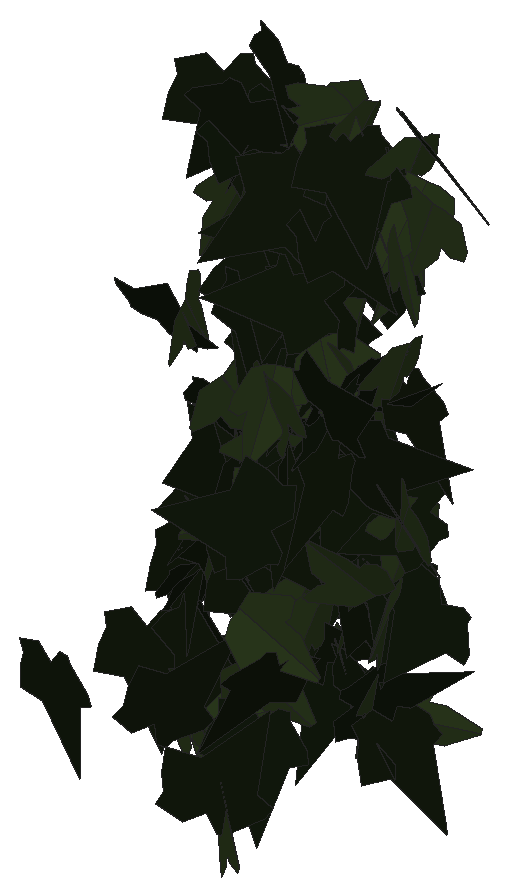
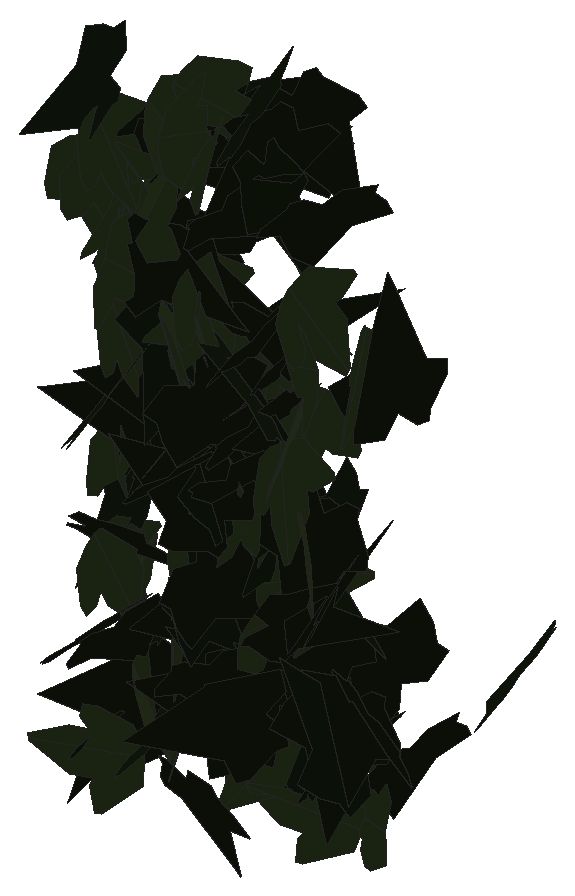
# SketchUp Ruby script. Lengths in inches.
U = 1.inch
M = Sketchup.active_model
def pt(a) = Geom::Point3d.new(a.map { |v| v * U })
def face(e, loops, mat)
  f = e.add_face(loops[0].map { |a| pt(a) })
  loops[1..].each { |l| e.add_face(l.map { |a| pt(a) }).erase! }
  f.material = f.back_material = mat if mat
  f
end
# faces: each face lists its corners as indices into pts; further lists are holes
def faces(e, pts, list, mat = nil) = list.each { |f| face(e, (f[0].is_a?(Array) ? f : [f]).map { |l| l.map { |i| pts[i] } }, mat) }
# xy, xz, yz: faces in a plane at the given z, y or x. An outline is a flat list of corners, or four numbers for a rectangle; further outlines are holes
def ring(l) = l.size == 4 ? [[l[0], l[1]], [l[2], l[1]], [l[2], l[3]], [l[0], l[3]]] : l.each_slice(2).to_a
def flat(e, list, mat, &to3) = list.each { |f| face(e, (f[0].is_a?(Array) ? f : [f]).map { |l| ring(l).map { |u, v| to3.(u, v) } }, mat) }
def xy(e, z, list, mat = nil) = flat(e, list, mat) { |x, y| [x, y, z] }
def xz(e, y, list, mat = nil) = flat(e, list, mat) { |x, z| [x, y, z] }
def yz(e, x, list, mat = nil) = flat(e, list, mat) { |y, z| [x, y, z] }
def lines(e, pts, list) = list.each { |a, b| e.add_line(pt(pts[a]), pt(pts[b])) }
# prism: a flat outline (further loops are holes) pulled along v
def prism(e, loops, v, mat = nil)
  f = face(e, loops, mat); d = Geom::Vector3d.new(v.map { |x| x * U })
  f.pushpull(f.normal.samedirection?(d) ? d.length : -d.length)
end
def box(e, o, s, mat = nil) = prism(e, [[o, [o[0] + s[0], o[1], o[2]], [o[0] + s[0], o[1] + s[1], o[2]], [o[0], o[1] + s[1], o[2]]]], [0, 0, s[2]], mat)
def at(x, y, z, deg = 0) = Geom::Transformation.translation(pt([x, y, z])) * Geom::Transformation.rotation(ORIGIN, Z_AXIS, deg.degrees)
def axes(o, x, y, z) = Geom::Transformation.new([*x, 0, *y, 0, *z, 0, *pt(o).to_a, 1])
def part(name) = M.definitions.add(name)
# library, detail: a bought-in or finely detailed component or shape, given as its bounding box
def library(name, o, s) = part(name).tap { |d| box(d.entities, o, s) }
def detail(e, o, s) = box(e.add_group.entities, o, s)
def put(e, d, t, mat = nil) = e.add_instance(d, t).tap { |i| i.material = mat if mat }
def group(e, t, mat = nil) = e.add_group.tap { |g| g.transformation = t; g.material = mat if mat }.entities
root = M.entities
M.materials.add("efeu1").color = [18, 25, 13]
M.materials.add("efeu2").color = [43, 57, 29]
c1 = part("ivyleaf_9")
p = [[1.54,2.16,1.25],[1.36,2.04,1.19],[-0.21,0.99,0.68],[-0.71,1.11,0.82],[-0.85,0.86,0.67],[-0.8,0.17,0.21],
  [-0.9,-0.01,0.1],[-0.67,-0.16,-0.02],[-0.08,-0.08,-0.05],[-0.03,-0.6,-0.4],[0.65,-0.88,-0.66],[0.83,-0.6,-0.49],
  [1.29,-0.42,-0.43],[1.8125,-0.07,-0.26],[1.21,0.44,0.15]]
faces(c1.entities,p,[[0,1,2,3,4,5,6,7,8,9,10,11,12,13,14]],"efeu1")
c2 = part("ivyleaf_10")
p = [[0,0.5,-0.03],[-0.0625,2.02,-0.43],[-0.19,2.01,-0.46],[-0.54,1.05,-0.29],[-0.52,0.625,-0.18],[-0.83,0.76,-0.28],
  [-1.16,0.64,-0.33],[-1.15,0.33,-0.24],[-0.77,-0.39,0.02],[-0.3,-0.51,0.16],[0.04,-0.48,0.23],[-0.02,2.01,-0.4375],
  [-0.06,2.01,-0.43],[0.04,-0.49,0.23],[0.67,-0.49,0.14],[1.38,0.36,-0.2],[1.375,0.51,-0.24],[0.81,0.65,-0.19],
  [0.62,0.59,-0.15],[0.6,1.09,-0.28],[0.5,1.23,-0.31]]
faces(c2.entities,p,[[0,1,2,3,4,5,6,7,8,9,10],[11,12,0,13,14,15,16,17,18,19,20]],"efeu2")
put(root,c1,axes([39.76,218.64,235.83],[-0.13606,0.27055,-0.39786],[0.04668,-0.40409,-0.29075],[-0.47886,-0.11626,0.0847]))
put(root,c1,axes([36.25,218.75,234.58],[0.18702,-0.45521,0.08836],[0.03479,-0.08123,-0.49213],[0.4624,0.19023,0.00129]))
put(root,c1,axes([39.43,218.87,237.54],[-0.20466,-0.00713,0.45614],[-0.39206,-0.25286,-0.17986],[0.23324,-0.43129,0.09792]))
put(root,c2,axes([38.78,218.87,233.33],[0.01309,-0.03717,0.49844],[0.43605,-0.24288,-0.02956],[0.24432,0.43546,0.02605]))
put(root,c2,axes([39.38,218.69,236.29],[0.21409,0.09828,0.44103],[0.40366,0.1777,-0.23555],[-0.20304,0.45691,-0.00325]))
put(root,c1,axes([38.51,218.92,233.37],[-0.26224,-0.03724,0.42408],[0.42523,0.00076,0.26302],[-0.02024,0.49861,0.03127]))
put(root,c1,axes([37.61,219.08,234.19],[-0.04947,-0.09741,0.48792],[0.43073,0.23704,0.091],[-0.24904,0.42933,0.06046]))
put(root,c1,axes([39.52,219.89,238.75],[0.00714,-0.088,0.49214],[0.33503,-0.36449,-0.07004],[0.37109,0.33076,0.05376]))
put(root,c1,axes([39.68,219.88,238.1],[-0.44399,0.06238,-0.22132],[0.21925,-0.0302,-0.44835],[-0.06931,-0.49517,-0.00053]))
put(root,c2,axes([39.91,220.1,236.36],[-0.40421,-0.08589,-0.28149],[-0.23076,-0.20433,0.3937],[-0.18266,0.44819,0.12554]))
put(root,c1,axes([37.66,220.07,236.33],[0.2605,-0.32329,0.27862],[0.18678,-0.20714,-0.41498],[0.38374,0.32028,0.01285]))
put(root,c1,axes([38.71,220.39,241.16],[-0.31078,-0.28387,0.26988],[-0.20949,-0.17063,-0.42071],[0.33095,-0.37457,-0.01288]))
put(root,c1,axes([38.23,220.25,233.8],[-0.06334,-0.49315,-0.05281],[0.00648,0.05242,-0.4972],[0.49593,-0.06367,-0.00025]))
put(root,c2,axes([38.35,220.33,238.47],[0.17904,0.42174,-0.20019],[-0.09684,-0.17619,-0.4578],[-0.45669,0.2027,0.01859]))
put(root,c1,axes([38.63,220.4375,237.36],[-0.349,-0.18893,-0.30415],[0.32579,0.00863,-0.37919],[0.14853,-0.46285,0.11707]))
put(root,c1,axes([36.36,220.42,234.37],[0.01984,-0.48648,-0.11377],[-0.01924,0.11303,-0.48668],[0.49924,0.02369,-0.01423]))
put(root,c1,axes([38.87,220.58,239.74],[-0.29959,-0.02659,0.39942],[-0.33646,-0.25359,-0.26924],[0.2169,-0.4301,0.13405]))
put(root,c1,axes([39.4,220.11,238.43],[-0.17276,0.42988,0.18803],[-0.08534,0.16824,-0.46305],[-0.46138,-0.19209,0.01525]))
put(root,c2,axes([38.4,220.3,238.44],[-0.45879,0.17255,0.09869],[-0.09876,0.01757,-0.48983],[-0.17251,-0.46895,0.01796]))
put(root,c1,axes([37.99,220.3,236.6875],[-0.05967,-0.17832,-0.46329],[0.17798,0.42792,-0.18763],[0.46343,-0.1873,0.0124]))
put(root,c2,axes([36.67,220.59,233.44],[0.02179,-0.1026,0.48887],[0.48921,-0.09452,-0.04165],[0.10097,0.48014,0.09627]))
put(root,c1,axes([38.72,220.76,240.77],[-0.31497,-0.10729,0.37321],[-0.32879,-0.182,-0.32981],[0.20662,-0.45317,0.0441]))
put(root,c1,axes([36.375,220.64,238.58],[0.49365,-0.07686,-0.02004],[0.02026,-0.00015,0.49959],[-0.0768,-0.49406,0.00297]))
put(root,c2,axes([39.67,220.93,235.59],[-0.13396,0.02209,-0.48121],[0.10821,-0.48533,-0.0524],[-0.46941,-0.11818,0.12525]))
put(root,c1,axes([36.93,220.95,234.24],[-0.09406,-0.44669,0.204],[-0.002,-0.20736,-0.45497],[0.49107,-0.0864,0.03722]))
put(root,c1,axes([37.76,220.71,235.64],[0.04044,-0.47239,-0.15879],[-0.01342,0.15822,-0.47412],[0.49818,0.04261,0.00012]))
put(root,c2,axes([38.54,220.85,235.16],[0.0001,-0.4324,0.25106],[0.07571,-0.24815,-0.42742],[0.49423,0.0381,0.06543]))
put(root,c1,axes([37.13,220.92,234.2],[0.05501,-0.20512,0.45266],[0.24457,-0.38528,-0.20431],[0.43262,0.24389,0.05794]))
put(root,c2,axes([38.18,220.67,237.43],[-0.41792,-0.26691,0.06405],[-0.04939,-0.04166,-0.49581],[0.27001,-0.42074,0.00846]))
put(root,c2,axes([37.63,221,236.17],[0.00677,-0.02501,0.49933],[-0.15615,-0.4745,-0.02164],[0.47494,-0.15565,-0.01423]))
put(root,c2,axes([36.9,220.51,238.99],[0.12288,-0.38521,-0.29414],[0.02475,0.30804,-0.39307],[0.48403,0.08204,0.09477]))
put(root,c1,axes([37.63,220.77,241.88],[0.14433,0.19089,-0.43901],[-0.24233,-0.36631,-0.23894],[-0.41285,0.28174,-0.01322]))
put(root,c2,axes([37.52,220.58,238.09],[-0.20547,-0.37433,-0.26011],[0.16813,0.20296,-0.4249],[0.42369,-0.26207,0.04247]))
put(root,c2,axes([37.41,220.41,235.96],[0.07698,-0.16348,-0.4662],[-0.00652,0.47145,-0.1664],[0.494,0.0317,0.07046]))
put(root,c1,axes([38.92,220.68,240.84],[0.21776,-0.3615,-0.26813],[-0.03657,0.28267,-0.4108],[0.4486,0.19853,0.09667]))
put(root,c1,axes([38.96,221.11,235.5],[0.04763,-0.30648,0.39217],[0.08264,-0.38362,-0.30984],[0.49082,0.09434,0.01411]))
put(root,c2,axes([37.17,220.625,233.3],[0.18953,-0.03808,-0.46111],[0.45175,0.12291,0.17554],[0.09998,-0.48316,0.081]))
put(root,c1,axes([37.37,220.88,236.59],[-0.40634,0.24107,-0.16361],[0.11579,-0.12404,-0.47033],[-0.26735,-0.42012,0.04498]))
put(root,c2,axes([38.86,220.72,238.85],[0.16076,0.46841,0.0689],[0.01678,0.06708,-0.4952],[-0.47315,0.16153,0.00585]))
put(root,c1,axes([39.03,221.15,237.29],[-0.11335,-0.46483,0.1452],[-0.03646,-0.14056,-0.47845],[0.48562,-0.11905,-0.00203]))
put(root,c1,axes([38.5,221,238.58],[-0.4439,0.06429,-0.22096],[0.20999,-0.08323,-0.44607],[-0.09414,-0.48881,0.04689]))
put(root,c1,axes([38.42,220.54,237.43],[0.16874,-0.01161,-0.47052],[-0.39558,0.26734,-0.14846],[0.25503,0.42236,0.08104]))
put(root,c1,axes([37.51,221.12,238.98],[0.06689,-0.48049,0.12108],[0.0066,-0.1213,-0.48502],[0.49546,0.06649,-0.00989]))
put(root,c2,axes([38.14,221.11,235.16],[-0.05033,-0.42618,0.25659],[0.04615,-0.26079,-0.4241],[0.49531,-0.01901,0.06559]))
put(root,c1,axes([37.65,221.1,236.71],[0.24905,-0.30701,0.30614],[0.17873,-0.24896,-0.39506],[0.395,0.30622,-0.01426]))
put(root,c2,axes([37.75,220.78,234.16],[-0.35852,-0.17582,-0.30092],[0.27155,0.12969,-0.3993],[0.21846,-0.44974,0.0025]))
put(root,c1,axes([38.41,220.9,237.67],[-0.39828,0.30186,-0.01598],[0.01187,-0.01079,-0.49974],[-0.30205,-0.39845,0.00143]))
put(root,c1,axes([37.375,220.79,235.7],[0.27858,0.3249,-0.25852],[-0.17991,-0.18612,-0.42778],[-0.3742,0.33136,0.01321]))
put(root,c1,axes([37.66,221.14,239.4],[-0.37858,-0.26699,-0.18813],[0.15865,0.10142,-0.46319],[0.28549,-0.4104,0.00792]))
put(root,c1,axes([39.18,220.64,238.6],[0.11541,0.46581,0.14036],[0.03415,0.13614,-0.47989],[-0.4853,0.12035,-0.00039]))
put(root,c2,axes([39.35,221.14,234.4375],[0.22315,-0.43437,0.10734],[0.03799,-0.10112,-0.48819],[0.44582,0.22604,-0.01212]))
put(root,c2,axes([38.68,220.93,238.83],[-0.45257,0.03297,0.20999],[-0.2084,0.02845,-0.45361],[-0.04186,-0.4981,-0.01201]))
put(root,c1,axes([38.84,221.02,239.51],[-0.22718,-0.00558,-0.44537],[-0.40969,-0.19354,0.21141],[-0.17476,0.46099,0.08337]))
put(root,c2,axes([38.93,220.83,237.95],[0.20368,-0.3132,-0.33229],[-0.05946,0.34256,-0.35933],[0.45274,0.1859,0.1023]))
put(root,c1,axes([38.89,221.17,241.58],[-0.0484,-0.47345,-0.1533],[0.03336,0.15059,-0.47561],[0.49653,-0.05627,0.01701]))
put(root,c1,axes([36.71,221.4375,236.34],[-0.13244,-0.15306,0.4572],[-0.09101,-0.45767,-0.17959],[0.47347,-0.13079,0.09337]))
put(root,c1,axes([39.01,220.7,237.78],[0.0449,0.43552,-0.24147],[0.02863,0.23979,0.43781],[0.49716,-0.05314,-0.00341]))
put(root,c1,axes([39.24,220.86,237.51],[0.28041,0.12475,-0.39472],[0.23591,0.34361,0.27619],[0.34017,-0.34113,0.13384]))
put(root,c1,axes([38.14,221.43,237.98],[-0.2051,-0.41027,0.19903],[-0.05302,-0.1953,-0.45722],[0.4529,-0.20866,0.0366]))
put(root,c1,axes([36.24,221.28,235.21],[-0.2201,-0.15996,-0.41949],[0.44187,0.00546,-0.23392],[0.07942,-0.47369,0.13896]))
put(root,c2,axes([38.48,221.47,236.52],[0.00304,-0.17379,0.46882],[0.02068,-0.46838,-0.17376],[0.49956,0.02045,0.00434]))
put(root,c1,axes([39.61,221.1,233.92],[0.15078,-0.41243,-0.2391],[-0.03401,0.24083,-0.43686],[0.47551,0.148,0.04457]))
put(root,c1,axes([37.5,220.94,241.6],[-0.02971,-0.1783,-0.46618],[0.11044,0.45308,-0.18033],[0.48674,-0.11369,0.01246]))
put(root,c2,axes([38.34,221.4,239.21],[0.21161,-0.27485,0.36011],[0.24173,-0.26764,-0.34632],[0.38313,0.32066,0.01961]))
put(root,c2,axes([39.94,221,236.99],[-0.34654,0.16045,0.32275],[-0.31072,0.09391,-0.38031],[-0.18266,-0.46415,0.03462]))
put(root,c2,axes([38.57,221.23,241.85],[0.21598,0.05612,-0.44744],[-0.44619,-0.04529,-0.22105],[-0.06534,0.49477,0.03052]))
put(root,c1,axes([38.875,221.28,241.26],[-0.25543,-0.34578,-0.25533],[0.17984,0.18379,-0.42881],[0.3904,-0.3109,0.03048]))
put(root,c1,axes([39.31,220.79,234.23],[0.0838,0.3238,-0.37166],[0.01843,0.37467,0.33058],[0.49258,-0.0691,0.05086]))
put(root,c2,axes([39,221.09,235.51],[0.20692,-0.40928,-0.19918],[-0.0342,0.2042,-0.45512],[0.45389,0.20197,0.05651]))
put(root,c1,axes([38.92,221.41,234.21],[0.16962,-0.43995,0.16636],[0.09797,-0.13992,-0.46992],[0.46003,0.19201,0.03873]))
put(root,c2,axes([39.54,221.32,238.84],[0.03635,-0.49022,0.09145],[0.00311,-0.09147,-0.49155],[0.49867,0.0363,-0.0036]))
put(root,c1,axes([37.61,221.55,238.32],[-0.08453,-0.47849,0.1179],[-0.01254,-0.11749,-0.48584],[0.49264,-0.08509,0.00787]))
put(root,c1,axes([37.91,221.1,234.62],[0.22992,0.15473,-0.41617],[0.30892,0.28088,0.2751],[0.31892,-0.38362,0.03356]))
put(root,c1,axes([37.67,221.0625,234.78],[-0.07026,-0.01442,0.49483],[0.48968,0.07135,0.0716],[-0.07268,0.49467,0.0041]))
put(root,c2,axes([38.41,221.4,239.61],[-0.01736,-0.48331,0.12692],[-0.00731,-0.12674,-0.48362],[0.49964,-0.01865,-0.00266]))
put(root,c1,axes([37.55,221.61,242.03],[0.07494,-0.38239,0.31331],[0.08685,-0.30178,-0.38909],[0.48666,0.11274,0.02119]))
put(root,c1,axes([37.96,221.1,235.8125],[0.12274,0.05753,-0.48127],[0.27075,0.40365,0.1173],[0.40203,-0.28941,0.06793]))
put(root,c1,axes([39.41,221.16,237],[0.43938,-0.09408,-0.21931],[-0.20968,0.06721,-0.44891],[0.11395,0.48645,0.0196]))
put(root,c2,axes([37.4,221.69,235.98],[-0.16037,-0.07212,0.46806],[0.15651,-0.47447,-0.01949],[0.44697,0.14027,0.17476]))
put(root,c1,axes([38.03,221.28,237.2],[0.1191,0.43922,0.20712],[-0.0669,-0.19638,0.45493],[0.48098,-0.13608,0.01199]))
put(root,c2,axes([38.33,221.32,241.35],[-0.1464,0.47013,-0.08686],[0.03136,-0.08121,-0.49236],[-0.47706,-0.14961,-0.00571]))
put(root,c2,axes([38.53,221.18,237.9],[-0.1059,0.14727,0.46594],[-0.46403,0.11913,-0.14312],[-0.15317,-0.46273,0.11144]))
put(root,c1,axes([36.4,221.2,234.56],[0.13626,0.4767,0.06474],[-0.02533,-0.06009,0.49573],[0.48041,-0.13838,0.00777]))
put(root,c2,axes([38.62,221.32,234.49],[-0.28661,0.4033,-0.07212],[0.04218,-0.05851,-0.49477],[-0.40752,-0.2897,-0.00048]))
put(root,c1,axes([37.77,221.68,237.67],[-0.28067,-0.40766,0.07098],[-0.05282,-0.04977,-0.49471],[0.4104,-0.2852,-0.01513]))
put(root,c1,axes([38.45,221.54,238.1],[0.21434,-0.45111,0.02359],[0.01047,-0.02114,-0.49944],[0.45161,0.21459,0.00039]))
put(root,c1,axes([36.64,221.14,235.09],[0.13227,0.48177,-0.02],[-0.00801,-0.01854,-0.49959],[-0.48212,0.13248,0.00281]))
put(root,c2,axes([38.72,221.64,241.7],[0.1102,-0.4208,0.24654],[0.04894,-0.24193,-0.43482],[0.48524,0.11997,-0.01213]))
put(root,c2,axes([38.41,221.79,241.61],[0.02894,-0.15375,0.47489],[0.1514,-0.45058,-0.1551],[0.47565,0.15277,0.02048]))
put(root,c1,axes([38.29,221.66,236.27],[-0.24736,0.21255,-0.37899],[0.21464,-0.31941,-0.31923],[-0.37782,-0.32062,0.06677]))
put(root,c2,axes([37.2,221.21,238.43],[0.20903,-0.29143,-0.34839],[0.04508,0.39493,-0.30332],[0.45197,0.0954,0.19138]))
put(root,c1,axes([39.1,221.59,239.96],[-0.01271,-0.01449,-0.49963],[-0.3546,-0.35198,0.01923],[-0.35228,0.35482,-0.00133]))
put(root,c2,axes([37.91,221.42,237.31],[-0.45909,0.17044,-0.10093],[0.09923,-0.02261,-0.48953],[-0.17143,-0.46951,-0.01307]))
put(root,c1,axes([37.45,221.48,241.41],[-0.26304,0.38496,-0.18059],[0.11511,-0.13996,-0.46601],[-0.40934,-0.28673,-0.01499]))
put(root,c1,axes([37.74,221.81,240.99],[-0.17205,-0.45489,0.11609],[-0.04747,-0.10615,-0.48629],[0.46706,-0.17835,-0.00666]))
put(root,c1,axes([38.09,221.78,236.59],[-0.10787,0.1086,-0.47599],[0.17035,-0.44846,-0.14093],[-0.45754,-0.19258,0.05975]))
put(root,c1,axes([36.84,221.32,237.38],[0.40103,0.20833,-0.21394],[-0.19176,-0.09495,-0.4519],[-0.22892,0.4445,0.00374]))
put(root,c2,axes([36.76,221.72,240.13],[-0.01202,-0.43401,0.24798],[-0.006,-0.24791,-0.43417],[0.49982,-0.01341,0.00075]))
put(root,c1,axes([38.4375,221.84,237.5625],[-0.17298,-0.45635,0.10874],[0.06207,-0.13714,-0.4768],[0.465,-0.15146,0.1041]))
put(root,c1,axes([39.63,221.92,235.21],[-0.208,-0.37651,0.25491],[0.01482,-0.28578,-0.41001],[0.45444,-0.16301,0.13004]))
put(root,c2,axes([39.47,221.74,240.82],[-0.36052,-0.25173,0.23803],[-0.05555,-0.29709,-0.39831],[0.34196,-0.31364,0.18625]))
put(root,c1,axes([37.96,221.76,235.4],[-0.2208,-0.43703,-0.10127],[0.05499,0.08565,-0.48953],[0.44522,-0.22731,0.01024]))
put(root,c1,axes([38.12,221.78,238.68],[-0.00348,0.10391,-0.48907],[-0.10282,-0.47878,-0.101],[-0.4893,0.09987,0.0247]))
put(root,c2,axes([39.41,221.5,240.27],[-0.11104,0.48739,-0.01121],[0.00233,-0.01096,-0.49987],[-0.48751,-0.11106,0.00016]))
put(root,c2,axes([38.61,221.64,239.1],[0.33745,-0.36871,-0.01323],[-0.00835,0.01029,-0.49982],[0.36886,0.33756,0.00079]))
put(root,c1,axes([37,221.91,236.3],[-0.31399,-0.23388,0.31098],[-0.25898,-0.17263,-0.39131],[0.29041,-0.40682,-0.01274]))
put(root,c2,axes([39.8,221.57,240.77],[-0.45867,-0.02053,0.19799],[-0.19345,-0.07115,-0.45554],[0.04688,-0.49449,0.05733]))
put(root,c2,axes([37.14,221.57,237.99],[-0.04013,-0.49261,-0.07567],[-0.00107,0.076,-0.49419],[0.49839,-0.0395,-0.00715]))
put(root,c1,axes([39.36,221.68,238.19],[0.24607,-0.43352,-0.0389],[-0.01092,0.03852,-0.49839],[0.43512,0.24613,0.00949]))
put(root,c1,axes([39.53,221.78,236.52],[-0.46777,0.03711,0.17268],[-0.17662,-0.09991,-0.45697],[0.00059,-0.48851,0.10658]))
put(root,c1,axes([39.14,221.88,235.51],[-0.11495,-0.48447,0.04553],[0.00059,-0.04692,-0.49779],[0.48661,-0.11439,0.01136]))
put(root,c1,axes([39.5,221.6,241.87],[0.43456,-0.24232,0.04941],[0.04218,-0.02581,-0.49755],[0.24369,0.43659,-0.00199]))
put(root,c2,axes([38.97,221.55,240.29],[-0.3809,0.27303,-0.17427],[-0.14992,0.08986,0.46846],[0.28712,0.40912,0.01341]))
put(root,c1,axes([38.27,221.75,233.88],[-0.45327,-0.04526,-0.20616],[0.20394,0.0319,-0.4554],[0.05437,-0.49692,-0.01046]))
put(root,c1,axes([37.3,221.89,239.61],[0.01971,-0.48708,0.11121],[0.02615,-0.11014,-0.48702],[0.49893,0.02501,0.02113]))
put(root,c1,axes([36.47,221.76,241.44],[-0.08583,-0.45423,-0.19054],[0.06456,0.18137,-0.46145],[0.48833,-0.10381,0.02752]))
put(root,c2,axes([39.3,221.87,236.34],[-0.0639,-0.44172,0.2254],[0.06588,-0.23281,-0.43756],[0.4915,-0.02622,0.08795]))
put(root,c2,axes([39.35,221.8125,241.38],[-0.03136,-0.47668,0.14763],[-0.00586,-0.14756,-0.47769],[0.49898,-0.03169,0.00367]))
put(root,c2,axes([39.35,221.58,233.78],[-0.03654,0.0154,-0.49843],[0.49813,0.02424,-0.03576],[0.02306,-0.49917,-0.01712]))
put(root,c2,axes([36.58,221.89,239.52],[-0.18456,0.14223,-0.44239],[0.2719,-0.35296,-0.22692],[-0.37684,-0.32433,0.05294]))
put(root,c2,axes([36.98,221.41,236.93],[-0.01006,0.05502,0.49686],[-0.4077,0.28667,-0.04],[-0.28927,-0.40595,0.03909]))
put(root,c1,axes([37.7,221.41,238.64],[-0.32854,0.37652,-0.01717],[-0.01823,0.00689,0.49962],[0.37647,0.32892,0.0092]))
put(root,c1,axes([37.57,221.44,234.83],[0.3572,0.10354,0.3342],[0.32217,0.08891,-0.37189],[-0.13643,0.48102,-0.0032]))
put(root,c2,axes([39.15,221.95,239.93],[-0.0629,0.31857,-0.38021],[-0.06635,-0.38521,-0.31179],[-0.49157,0.01123,0.09073]))
put(root,c1,axes([37.93,221.66,237.18],[0.07078,-0.05639,0.49174],[0.47451,-0.13361,-0.08362],[0.14083,0.47851,0.0346]))
